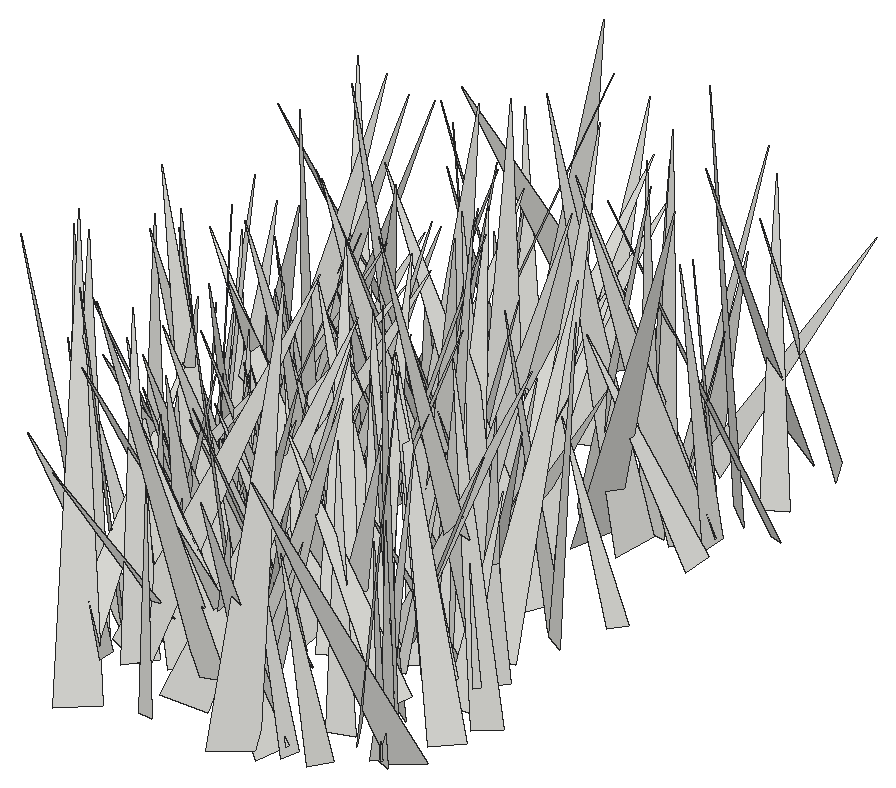
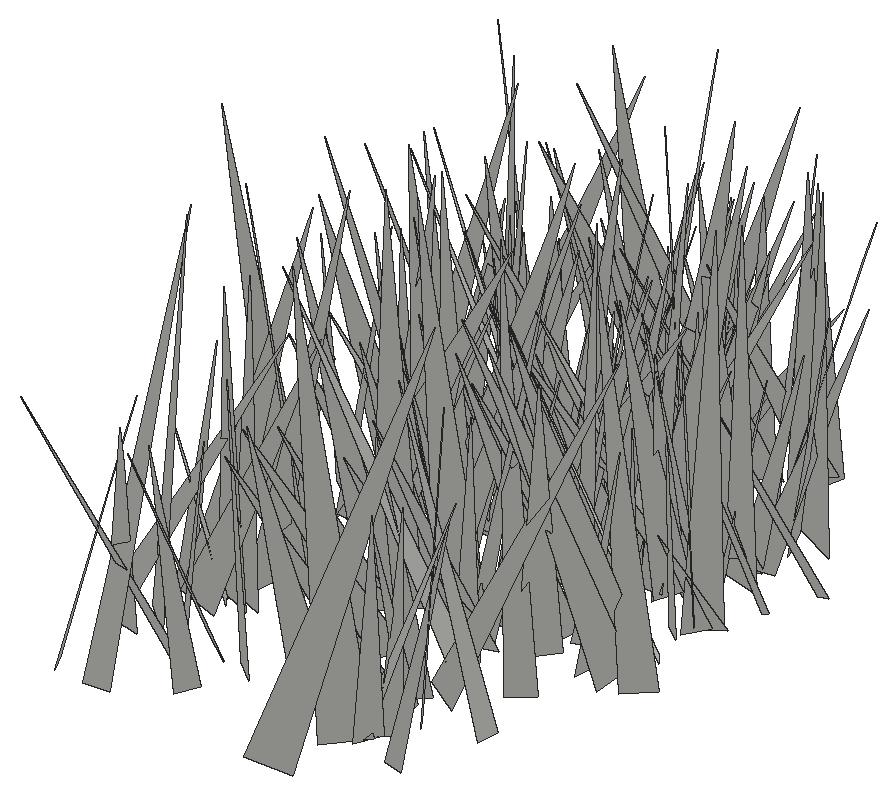
# SketchUp Ruby script. Lengths in inches.
U = 1.inch
M = Sketchup.active_model
def pt(a) = Geom::Point3d.new(a.map { |v| v * U })
def face(e, loops, mat)
  f = e.add_face(loops[0].map { |a| pt(a) })
  loops[1..].each { |l| e.add_face(l.map { |a| pt(a) }).erase! }
  f.material = f.back_material = mat if mat
  f
end
# faces: each face lists its corners as indices into pts; further lists are holes
def faces(e, pts, list, mat = nil) = list.each { |f| face(e, (f[0].is_a?(Array) ? f : [f]).map { |l| l.map { |i| pts[i] } }, mat) }
# xy, xz, yz: faces in a plane at the given z, y or x. An outline is a flat list of corners, or four numbers for a rectangle; further outlines are holes
def ring(l) = l.size == 4 ? [[l[0], l[1]], [l[2], l[1]], [l[2], l[3]], [l[0], l[3]]] : l.each_slice(2).to_a
def flat(e, list, mat, &to3) = list.each { |f| face(e, (f[0].is_a?(Array) ? f : [f]).map { |l| ring(l).map { |u, v| to3.(u, v) } }, mat) }
def xy(e, z, list, mat = nil) = flat(e, list, mat) { |x, y| [x, y, z] }
def xz(e, y, list, mat = nil) = flat(e, list, mat) { |x, z| [x, y, z] }
def yz(e, x, list, mat = nil) = flat(e, list, mat) { |y, z| [x, y, z] }
def lines(e, pts, list) = list.each { |a, b| e.add_line(pt(pts[a]), pt(pts[b])) }
# prism: a flat outline (further loops are holes) pulled along v
def prism(e, loops, v, mat = nil)
  f = face(e, loops, mat); d = Geom::Vector3d.new(v.map { |x| x * U })
  f.pushpull(f.normal.samedirection?(d) ? d.length : -d.length)
end
def box(e, o, s, mat = nil) = prism(e, [[o, [o[0] + s[0], o[1], o[2]], [o[0] + s[0], o[1] + s[1], o[2]], [o[0], o[1] + s[1], o[2]]]], [0, 0, s[2]], mat)
def at(x, y, z, deg = 0) = Geom::Transformation.translation(pt([x, y, z])) * Geom::Transformation.rotation(ORIGIN, Z_AXIS, deg.degrees)
def axes(o, x, y, z) = Geom::Transformation.new([*x, 0, *y, 0, *z, 0, *pt(o).to_a, 1])
def part(name) = M.definitions.add(name)
# library, detail: a bought-in or finely detailed component or shape, given as its bounding box
def library(name, o, s) = part(name).tap { |d| box(d.entities, o, s) }
def detail(e, o, s) = box(e.add_group.entities, o, s)
def put(e, d, t, mat = nil) = e.add_instance(d, t).tap { |i| i.material = mat if mat }
def group(e, t, mat = nil) = e.add_group.tap { |g| g.transformation = t; g.material = mat if mat }.entities
root = M.entities
c1 = part("fur_instance\#9")
p = [[0.8125,0,1.79],[0.67,-0.02,1.48],[0,-0.11,0],[0,0.11,0]]
faces(c1.entities,p,[[0,1,2,3]])
put(root,c1,axes([99.53,207.82,-27.1],[-3.854,-0.48704,1.31581],[-0.33639,4.05498,0.51565],[1.36213,-0.37663,3.85028]))
put(root,c1,axes([100.16,194.93,-28.22],[1.87849,6.8023,2.53671],[7.02619,-2.36292,1.13321],[-1.82724,-2.09291,6.96533]))
put(root,c1,axes([100.67,195.38,-28.22],[-4.99068,-1.45127,1.21381],[-1.71677,4.91279,-1.18474],[0.79513,1.49823,5.06058]))
put(root,c1,axes([99.54,205.16,-28.22],[2.36348,3.65871,1.87372],[3.9267,-2.64879,0.21906],[-1.21573,-1.4425,4.3502]))
put(root,c1,axes([102.27,193.58,-27.1],[-6.74391,-2.32387,0.77011],[-2.44649,6.31426,-2.37034],[-0.09,2.49068,6.72772]))
put(root,c1,axes([98.67,206.66,-27.1],[6.0321,-2.57805,3.10449],[-3.62742,-5.91038,2.14001],[-1.76807,3.33038,6.20104]))
put(root,c1,axes([97.26,207.74,-27.1],[1.41766,-6.83451,0.48866],[-6.53171,-1.19719,2.20513],[2.07029,0.90294,6.62252]))
put(root,c1,axes([98.46,207.52,-27.1],[6.56769,-0.93589,1.93904],[-1.50422,-6.44796,1.98276],[-1.54048,2.30611,6.3308]))
put(root,c1,axes([99.47,201.66,-28.22],[6.10585,-2.9623,2.45846],[-2.96929,-6.55789,-0.52733],[-2.45002,0.56525,6.76598]))
put(root,c1,axes([101.33,207.83,-27.1],[-5.19034,4.80556,0.45379],[4.78626,5.21014,-0.43029],[0.62529,0.00866,7.0603]))
put(root,c1,axes([100.43,197.4,-28.22],[3.46257,-3.0651,1.27719],[-2.41097,-3.5895,-2.07802],[-2.28326,-0.85797,4.13111]))
put(root,c1,axes([102.11,211.93,-27.1],[-3.14306,-6.22127,0.26286],[-6.12359,3.03481,-1.39417],[-1.12913,0.859,6.8293]))
put(root,c1,axes([100.4,198.49,-28.22],[1.00735,6.64791,2.58508],[7.07427,-1.26504,0.49655],[-0.91221,-2.46923,6.70544]))
put(root,c1,axes([100.78,197.67,-28.22],[-2.91756,2.69263,1.56889],[3.08399,2.80363,0.92331],[0.448,-1.76443,3.86133]))
put(root,c1,axes([100.94,194.41,-27.1],[-0.82841,6.75025,1.93378],[7.00258,0.65031,0.72978],[-0.51887,-2.00072,6.76162]))
put(root,c1,axes([100.41,216.59,-27.1],[-1.40933,-4.17013,0.64925],[-4.20295,1.44894,0.18319],[0.38311,0.55526,4.39803]))
put(root,c1,axes([100.12,202.41,-28.22],[2.1369,3.02619,1.55246],[3.28055,-2.31782,0.00255],[-0.89775,-1.26656,3.70461]))
put(root,c1,axes([101.0625,199.84,-28.22],[2.9038,6.51052,1.10748],[6.2299,-3.10193,1.9005],[-2.1913,-0.1914,6.87074]))
put(root,c1,axes([100.12,201.24,-28.22],[-3.74017,-2.83655,2.38458],[-3.12746,4.23356,0.13062],[1.98777,1.32365,4.69232]))
put(root,c1,axes([102.41,191.93,-28.22],[-7.32021,3.8589,0.48336],[3.73123,7.2592,-1.44642],[1.09666,1.05977,8.14767]))
put(root,c1,axes([100.45,201.95,-27.1],[-4.55508,3.55475,2.05706],[3.40532,4.98624,-1.07596],[2.29598,-0.34303,5.67691]))
put(root,c1,axes([101.89,200.34,-28.22],[-5.70534,2.42628,0.74712],[2.22137,5.6608,-1.42016],[1.22905,1.03174,6.03498]))
put(root,c1,axes([100.52,199.53,-28.22],[-3.02452,-1.82217,1.01563],[-1.34667,3.07159,1.50047],[1.5932,-0.86291,3.19635]))
put(root,c1,axes([102.8,214.93,-27.1],[-4.27144,-3.27285,0.83505],[-3.36103,3.98484,-1.57435],[-0.33515,1.75031,5.14569]))
put(root,c1,axes([100.61,198.03,-28.22],[-0.48959,-3.44443,1.08487],[-3.54488,0.6673,0.51889],[0.68909,0.98557,3.44014]))
put(root,c1,axes([98.13,205.59,-27.1],[4.83025,3.81866,0.07193],[3.65702,-4.5907,-1.86288],[1.10161,-1.50398,5.86882]))
put(root,c1,axes([101.55,195.35,-27.1],[-4.35453,-4.53446,2.05004],[-4.74623,4.60317,0.10013],[1.49574,1.4055,6.28595]))
put(root,c1,axes([100.39,206.33,-27.1],[5.08436,-3.96797,0.13679],[-3.71243,-4.83007,-2.12193],[-1.40762,-1.5937,6.0904]))
put(root,c1,axes([100.04,205.7,-27.1],[7.02888,1.27959,1.54515],[0.73768,-6.88381,2.34499],[-1.86566,2.099,6.7486]))
put(root,c1,axes([101.61,201.23,-27.1],[2.47706,-6.70826,1.39737],[-6.69174,-2.68793,-1.04158],[-1.47445,0.92925,7.07472]))
put(root,c1,axes([99.2,206.34,-27.1],[-0.29614,5.30233,1.4786],[4.87042,0.94241,-2.40408],[2.56516,-1.17721,4.73528]))
put(root,c1,axes([102.18,215.67,-27.1],[-4.07522,2.66076,1.05763],[2.66001,4.19896,-0.31421],[1.05952,-0.30776,4.85678]))
put(root,c1,axes([98.56,199.53,-28.22],[3.67258,4.04026,0.63824],[3.75616,-2.99162,-2.6759],[1.61937,-2.22383,4.75932]))
put(root,c1,axes([97.76,197.5,-28.22],[4.06376,5.39951,0.02576],[4.83357,-3.62337,-3.0294],[2.40665,-1.8401,6.04083]))
put(root,c1,axes([101.64,213.56,-27.1],[-4.27511,-3.26782,2.05551],[-3.38668,4.64678,0.34365],[1.85313,0.95347,5.37002]))
put(root,c1,axes([102.23,204.49,-28.22],[-3.60643,-6.53276,3.39182],[-7.2869,3.70246,-0.61691],[1.0404,3.28673,7.43658]))
put(root,c1,axes([99.24,213.11,-27.1],[6.07626,0.90493,0.17774],[0.92213,-5.94508,-1.25588],[0.01299,-1.26833,6.01354]))
put(root,c1,axes([100.4375,198.77,-27.1],[2.54415,-5.74451,1.38415],[-5.89364,-2.3587,1.04378],[0.42454,1.68081,6.19537]))
put(root,c1,axes([102.03,200.9,-27.1],[3.56835,-1.26097,2.05366],[-1.59686,-3.9854,0.32755],[-1.80488,1.03305,3.77039]))
put(root,c1,axes([105.05,198.42,-28.22],[-4.54236,-5.48641,0.31776],[-5.31376,4.27953,-2.06985],[-1.40202,1.55551,6.81539]))
put(root,c1,axes([101.58,192.82,-27.1],[-1.51981,5.35977,0.02073],[5.22969,1.48762,-1.21441],[1.17387,0.31183,5.43711]))
put(root,c1,axes([102.57,200.48,-27.1],[3.27442,-5.47757,0.11686],[-5.10679,-3.10069,-2.24625],[-1.98447,-1.05885,5.97327]))
put(root,c1,axes([100.9375,203.56,-27.1],[2.11868,-4.0714,0.72457],[-4.11944,-2.00647,0.77101],[0.3627,0.99394,4.52445]))
put(root,c1,axes([101.58,200.22,-27.1],[3.83893,-0.81047,1.08867],[-0.8917,-3.9684,0.19003],[-1.0232,0.41758,3.91895]))
put(root,c1,axes([101.18,202.21,-27.1],[-2.08812,-6.42397,1.05341],[-6.15561,2.30841,1.87538],[2.11792,0.37569,6.48927]))
put(root,c1,axes([101.77,215.03,-27.1],[3.2467,-2.02133,0.75684],[-1.94033,-3.33216,-0.57574],[-0.94537,-0.10279,3.78092]))
put(root,c1,axes([103.27,203.58,-27.1],[-3.89447,-3.70378,1.65585],[-4.00703,3.87088,-0.766],[0.63525,1.71028,5.3196]))
put(root,c1,axes([102.22,213.4375,-27.1],[3.63401,0.67625,1.41653],[0.37628,-3.84346,0.86953],[-1.5239,0.6636,3.59267]))
put(root,c1,axes([101.24,199.92,-28.22],[5.91646,3.40669,0.5347],[3.12979,-5.75065,2.00759],[-1.44773,1.49011,6.52531]))
put(root,c1,axes([101.53,197.16,-28.22],[-0.19463,-4.95849,1.24268],[-5.00803,0.4343,0.94858],[1.02496,1.18047,4.8708]))
put(root,c1,axes([104.27,207.44,-27.1],[-7.25051,-1.24633,1.39987],[-1.43303,7.2913,-0.93068],[1.20805,1.16894,7.29774]))
put(root,c1,axes([99.125,201.36,-28.22],[2.23337,6.49328,0.05356],[5.9184,-2.0122,-2.84202],[2.67172,-0.9705,6.25089]))
put(root,c1,axes([100.08,210.36,-27.1],[-0.39765,-7.51588,0.89638],[-7.02687,0.7002,2.75371],[2.81337,0.68655,7.00455]))
put(root,c1,axes([104.01,203.61,-27.1],[-0.12405,-5.8754,2.10648],[-6.00776,-0.4589,-1.63376],[-1.69244,2.05962,5.64504]))
put(root,c1,axes([104.07,198.35,-28.22],[0.25275,3.74041,1.98428],[3.79537,-1.08135,1.55493],[-1.87703,-1.68284,3.41127]))
put(root,c1,axes([103.41,193.92,-27.1],[-5.08391,3.17186,1.29588],[3.17676,5.23223,-0.34381],[1.28383,-0.38638,5.98237]))
put(root,c1,axes([102.92,197.95,-27.1],[-0.42877,3.87256,1.55947],[4.17346,0.35848,0.25729],[-0.1042,-1.57711,3.88772]))
put(root,c1,axes([104.36,197.49,-27.1],[-1.56968,-5.60909,0.11931],[-5.50885,1.51747,-1.1357],[-1.06238,0.41882,5.71278]))
put(root,c1,axes([106.45,200.89,-27.1],[-3.37764,5.82202,0.02709],[5.22944,3.02002,2.9728],[-2.55923,-1.51283,6.03878]))
put(root,c1,axes([104.73,196.54,-27.1],[-3.07753,7.46975,2.03134],[7.70521,2.74591,1.57617],[-0.74375,-2.46119,7.92363]))
put(root,c1,axes([103.76,198.47,-28.22],[-4.72142,-2.258,0.83052],[-2.14472,4.77905,0.80066],[1.09019,-0.37724,5.17198]))
put(root,c1,axes([104.77,194.54,-27.1],[-1.73609,5.26171,0.91511],[5.1615,1.40586,1.70864],[-1.37182,-1.3693,5.27069]))
put(root,c1,axes([101.43,206.43,-27.1],[5.10289,-1.83511,1.25864],[-2.13691,-4.91957,1.49087],[-0.62081,1.84972,5.21387]))
put(root,c1,axes([105.28,195.8,-28.22],[-0.91918,-4.72146,0.08029],[-4.18667,0.777,-2.23865],[-2.18412,0.49761,4.25741]))
put(root,c1,axes([103.34,208.12,-27.1],[-1.39577,-4.42794,0.41329],[-4.44248,1.40819,0.08395],[0.20461,0.36877,4.64196]))
put(root,c1,axes([101.45,199.2,-28.22],[4.36053,2.62617,0.62372],[2.69593,-4.29581,-0.7602],[-0.13318,-0.97427,5.03319]))
put(root,c1,axes([101.8,207.12,-27.1],[3.71055,0.76796,0.33165],[0.80764,-3.68168,-0.51076],[-0.21789,-0.56867,3.7546]))
put(root,c1,axes([103.62,219.07,-27.1],[3.75973,-6.87339,0.18092],[-6.4988,-3.61971,-2.46477],[-2.2454,-1.03249,7.43666]))
put(root,c1,axes([102.93,198.07,-28.22],[5.9616,4.7587,3.0284],[5.08757,-6.43918,0.10304],[-2.43578,-1.80245,7.62727]))
put(root,c1,axes([102.84,195.16,-27.1],[4.75143,0.92242,1.33841],[0.70934,-4.89704,0.85681],[-1.46255,0.62163,4.7637]))
put(root,c1,axes([102.83,209.74,-27.1],[3.43508,-2.31671,0.74566],[-2.27877,-3.51457,-0.42176],[-0.85461,0.05948,4.12177]))
put(root,c1,axes([103.88,198.78,-28.22],[1.78326,-6.33726,0.7797],[-6.26284,-1.89367,-1.06754],[-1.24322,0.44943,6.49625]))
put(root,c1,axes([103.3,197.05,-27.1],[2.16413,-4.87719,1.14426],[-4.95965,-2.26151,-0.2591],[-0.70577,0.93721,5.32947]))
put(root,c1,axes([104.68,199.7,-28.22],[2.20766,-6.15742,1.48059],[-5.96151,-2.54967,-1.71445],[-2.13691,0.75174,6.31254]))
put(root,c1,axes([104.7,195.52,-28.22],[-3.64875,-2.02244,1.121],[-2.25149,3.58457,-0.86132],[0.52696,1.3118,4.08188]))
put(root,c1,axes([103.02,208.6,-27.1],[-0.26942,5.43204,0.24352],[5.36362,0.30555,-0.88154],[0.89325,-0.19629,5.36679]))
put(root,c1,axes([104.49,192.81,-28.22],[1.15906,3.62365,1.13013],[3.60388,-1.42153,0.86183],[-1.19166,-0.77453,3.7056]))
put(root,c1,axes([102.61,212.53,-27.1],[1.94389,-4.04886,0.80465],[-4.08173,-1.75236,1.04312],[0.61659,1.16421,4.36851]))
put(root,c1,axes([104.93,201.1,-28.22],[-5.52274,-3.05851,1.02558],[-2.84433,5.57616,1.31266],[1.52186,-0.67738,6.17511]))
put(root,c1,axes([103.68,202.9,-27.1],[3.85077,0.95797,1.10657],[0.6489,-3.90916,1.12606],[-1.31192,0.87829,3.80501]))
put(root,c1,axes([103.48,200.92,-27.1],[-2.78361,3.37072,1.19614],[3.02117,3.0272,-1.49988],[1.91443,0.12385,4.10617]))
put(root,c1,axes([103.35,209.32,-27.1],[-3.61899,-3.55384,3.43713],[-4.24844,4.41399,0.09065],[2.52873,2.32973,5.07136]))
put(root,c1,axes([105.98,194.57,-27.1],[-1.13695,-6.80591,1.9758],[-6.92615,0.64332,-1.76957],[-1.50086,2.18691,6.66945]))
put(root,c1,axes([102.68,216.23,-27.1],[5.49312,-5.94068,1.74056],[-6.16398,-5.4638,0.80479],[-0.57141,1.8305,8.05098]))
put(root,c1,axes([105.45,199.26,-27.1],[-1.01525,-4.25558,0.24661],[-4.20456,0.95799,-0.77812],[-0.70176,0.41691,4.30525]))
put(root,c1,axes([103.39,206.96,-27.1],[5.19652,-2.78136,0.42044],[-2.54268,-5.02221,-1.79688],[-1.20313,-1.39929,5.61347]))
put(root,c1,axes([104.83,197.23,-27.1],[-2.5051,-3.46967,0.23869],[-3.39401,2.50314,0.76559],[0.75915,-0.25846,4.21047]))
put(root,c1,axes([105.66,200.01,-27.1],[-2.79772,3.91125,0.86225],[4.00509,2.73873,0.57209],[0.02536,-1.03446,4.77471]))
put(root,c1,axes([105.96,207.42,-27.1],[-3.1075,-6.9448,0.74353],[-6.98342,3.07514,-0.46373],[-0.12218,0.86773,7.5942]))
put(root,c1,axes([102.39,210.39,-27.1],[7.40183,3.33475,0.3809],[3.31775,-7.40888,0.39208],[-0.5081,0.20159,8.10888]))
put(root,c1,axes([104.03,208.39,-27.1],[-3.12669,6.25889,3.83958],[6.87271,3.96367,-0.86451],[2.58493,-2.9678,6.9428]))
put(root,c1,axes([105.55,201.92,-28.22],[-3.08604,-1.58363,1.00431],[-1.62158,3.22493,0.10239],[0.94181,0.36349,3.46714]))
put(root,c1,axes([106.84,198.65,-27.1],[-4.54566,0.43172,0.55069],[0.54174,4.46219,0.97364],[0.44289,-1.02717,4.4611]))
put(root,c1,axes([102.85,194.11,-27.1],[1.48421,7.77893,1.22221],[7.56365,-1.06243,-2.42301],[2.19017,-1.60247,7.53948]))
put(root,c1,axes([109.28,193.46,-28.22],[-2.18408,5.95276,0.46734],[5.01759,1.55993,3.57972],[-3.2369,-1.59851,5.23366]))
put(root,c1,axes([102.64,199.72,-27.1],[1.86343,6.88556,0.79652],[6.51007,-1.45535,-2.64927],[2.37997,-1.41024,6.62304]))
put(root,c1,axes([105.21,206.23,-27.1],[4.98467,2.72403,1.68688],[2.57744,-5.26236,0.88159],[-1.90334,0.00786,5.61161]))
put(root,c1,axes([106.95,194.92,-27.1],[-6.4254,-4.61842,2.37343],[-5.01235,6.50279,-0.91585],[1.35622,2.15235,7.85982]))
put(root,c1,axes([104.47,201.32,-28.22],[4.44163,5.80553,0.93246],[5.82565,-4.50337,0.28854],[-0.79717,-0.56325,7.30404]))
put(root,c1,axes([105.65,214.26,-27.1],[-4.4871,3.83069,1.41429],[3.5666,4.69982,-1.41404],[1.98841,0.2144,5.72789]))
put(root,c1,axes([105.81,200.99,-28.22],[-0.46017,-7.01963,1.64197],[-7.20868,0.46604,-0.02793],[0.07879,1.64032,7.03464]))
put(root,c1,axes([104.03,197.22,-27.1],[3.98681,-3.04122,0.56389],[-3.08769,-3.85909,1.01744],[0.18196,1.14894,4.91004]))
put(root,c1,axes([105.97,199.24,-28.22],[-2.87377,-5.9267,0.11201],[-5.79461,2.83495,1.33509],[1.24935,-0.48389,6.44995]))
put(root,c1,axes([104.33,212.59,-27.1],[-1.05033,5.0969,0.69056],[4.61293,1.24522,-2.17458],[2.27512,-0.17172,4.72788]))
put(root,c1,axes([105.11,210.84,-27.1],[-2.16647,5.60636,0.16983],[5.26617,2.09582,-2.00715],[1.93067,0.57445,5.66535]))
put(root,c1,axes([107.71,204.57,-27.1],[2.58278,-6.81445,2.81399],[-6.72051,-3.40212,-2.07037],[-3.03151,1.73634,6.98721]))
put(root,c1,axes([106.48,196.6,-28.22],[2.5877,-3.76016,0.15432],[-3.53923,-2.49522,-1.45139],[-1.27925,-0.70276,4.32764]))
put(root,c1,axes([105.9375,196.74,-28.22],[4.8135,2.02359,1.54657],[1.94555,-5.05552,0.55956],[-1.64367,-0.05793,5.19149]))
put(root,c1,axes([104.54,196.76,-28.22],[6.50661,-0.43072,0.76621],[-0.39332,-6.54513,-0.33931],[-0.78607,-0.29036,6.51202]))
put(root,c1,axes([107.4375,197.33,-27.1],[-4.91949,-2.25789,1.34677],[-2.33985,5.06309,-0.05864],[1.19873,0.61667,5.41258]))
put(root,c1,axes([108.43,200.8,-28.22],[-3.37701,5.49526,1.43426],[5.6473,3.0721,1.52623],[-0.60248,-2.00587,6.26679]))
put(root,c1,axes([105.73,195.26,-27.1],[2.79472,-2.37927,0.19168],[-2.37504,-2.80125,-0.14262],[-0.23842,0.01542,3.66757]))
put(root,c1,axes([106.1,206.95,-27.1],[4.26152,0.65659,1.09682],[0.47447,-4.35714,0.76482],[-1.18701,0.6156,4.24343]))
put(root,c1,axes([104.97,194.25,-28.22],[-3.36255,6.42423,2.20976],[5.77924,4.00105,-2.8377],[3.57129,-0.42595,6.67271]))
put(root,c1,axes([108.16,198.3,-27.1],[-2.69969,6.39263,0.77147],[6.43614,2.65406,0.5304],[-0.19237,-0.91623,6.91901]))
put(root,c1,axes([106.88,208.33,-27.1],[4.92232,-5.34816,3.43981],[-5.97476,-5.37881,0.1869],[-2.17654,2.67018,7.26616]))
put(root,c1,axes([108.22,204.24,-27.1],[-4.1053,-4.23157,0.31859],[-4.21802,4.11764,0.33835],[0.46467,-0.00766,5.88602]))
put(root,c1,axes([111.23,204.73,-27.1],[-3.57057,6.8988,1.02898],[6.50769,2.8788,3.28081],[-2.51043,-2.34953,7.04122]))
put(root,c1,axes([108.18,200.41,-27.1],[2.13883,-4.28297,3.06723],[-5.00629,-2.68295,-0.2554],[-1.63976,2.60467,4.7805]))
put(root,c1,axes([107.53,195.35,-28.22],[1.37303,-5.10418,0.31363],[-5.09334,-1.39399,-0.38851],[-0.45708,0.20095,5.27134]))
put(root,c1,axes([106.73,205.19,-28.22],[6.65936,-3.07974,1.86174],[-3.09449,-6.89952,-0.34452],[-1.83712,0.458,7.32893]))
put(root,c1,axes([106.79,196,-27.1],[3.4607,5.10853,1.2476],[5.25066,-3.43918,-0.48234],[-0.29016,-1.30574,6.15149]))
put(root,c1,axes([107.52,208.44,-27.1],[-1.55041,4.4226,0.08121],[4.26043,1.51619,-1.23272],[1.18941,0.33394,4.52145]))
put(root,c1,axes([106.1875,196.55,-28.22],[4.99795,-3.82327,1.26682],[-4.01963,-4.86241,1.18375],[-0.25457,1.71502,6.18026]))
put(root,c1,axes([109.75,204.97,-27.1],[-3.22494,-3.97651,0.65226],[-4.0077,3.07801,-1.05003],[-0.42001,1.16258,5.01102]))
put(root,c1,axes([108.18,192.79,-28.22],[5.95771,-4.00613,4.25574],[-5.13988,-6.48421,1.09155],[-2.78246,3.40011,7.09591]))
put(root,c1,axes([109.43,201.05,-28.22],[-1.2405,4.10694,0.41743],[4.03089,1.11105,1.04764],[-0.89058,-0.69186,4.16031]))
put(root,c1,axes([108.11,204.12,-27.1],[-3.37958,0.77927,1.41196],[0.41341,3.58754,-0.99047],[1.55884,0.73803,3.32382]))
put(root,c1,axes([108.17,214.62,-27.1],[3.30572,4.13092,2.03155],[4.38871,-3.58299,0.14433],[-1.38957,-1.489,5.28881]))
put(root,c1,axes([108.15,200.93,-27.1],[3.13012,3.09581,1.75638],[3.35561,-3.34662,-0.08138],[-1.18695,-1.29717,4.40172]))
put(root,c1,axes([109.8125,193.71,-28.22],[-4.0966,0.35691,0.30901],[0.31396,4.07547,-0.54495],[0.35257,0.51784,4.07585]))
put(root,c1,axes([107.12,199.87,-27.1],[5.77926,4.78065,0.80242],[4.74367,-5.8345,0.5954],[-0.99801,-0.04845,7.47663]))
put(root,c1,axes([109.32,198.22,-27.1],[-1.91608,6.79372,1.10059],[6.8739,1.94553,-0.04218],[0.33984,-1.04766,7.05863]))
put(root,c1,axes([106.38,200.84,-27.1],[5.98331,3.57339,0.75673],[3.63565,-5.68637,-1.89446],[0.35186,-2.00943,6.70672]))
put(root,c1,axes([107.81,199.1,-27.1],[2.67886,-4.09104,0.57639],[-4.11516,-2.58128,0.80469],[0.36641,0.91951,4.82342]))
put(root,c1,axes([109.16,201.91,-28.22],[-5.34624,-2.21651,3.3319],[-3.00843,5.89263,-0.90721],[2.6389,2.22728,5.71596]))
put(root,c1,axes([111.65,196.98,-27.1],[-4.58774,2.19144,0.09862],[2.15217,4.45217,1.18567],[-0.42461,-1.11142,4.94408]))
put(root,c1,axes([109.84,214.01,-27.1],[2.78013,5.13783,0.11647],[4.85085,-2.66723,1.86951],[-1.69707,0.79284,5.53456]))
put(root,c1,axes([110.23,195.85,-28.22],[-0.93822,4.8343,1.08723],[4.93478,0.81164,0.64956],[-0.44769,-1.18472,4.88147]))
put(root,c1,axes([111.18,209.96,-27.1],[-8.03417,0.61584,1.78735],[0.70083,8.21761,0.3188],[1.75577,-0.4621,8.05143]))
put(root,c1,axes([112.21,212.03,-27.1],[-0.7555,-5.85213,2.53673],[-5.87032,-0.36099,-2.58111],[-2.49433,2.62211,5.30623]))
put(root,c1,axes([110.76,205,-27.1],[0.70826,8.01559,0.32411],[7.89046,-0.75477,1.42384],[-1.44754,-0.19233,7.91985]))
put(root,c1,axes([108.82,216.8,-27.1],[3.79566,-1.87078,0.73995],[-1.92959,-3.83243,0.2087],[-0.56925,0.51676,4.2265]))
put(root,c1,axes([110.46,198.67,-27.1],[1.53322,3.39,0.04746],[3.12816,-1.43461,1.41479],[-1.30727,0.54307,3.44111]))
put(root,c1,axes([110.29,200.85,-28.22],[2.96295,7.07925,2.39249],[7.30087,-3.29107,0.69644],[-1.59283,-1.91622,7.64263]))
put(root,c1,axes([110.62,214.79,-27.1],[-2.70575,-2.79772,1.42447],[-3.05403,2.78134,-0.3384],[0.7275,1.27058,3.87735]))
put(root,c1,axes([108.43,203.74,-27.1],[2.40948,7.1196,1.80641],[7.28749,-2.07931,-1.52526],[0.91887,-2.17835,7.35989]))
put(root,c1,axes([111.09,200.8,-28.22],[-5.51425,5.90533,1.65371],[5.90522,5.71303,-0.71018],[1.6541,-0.70927,8.04832]))
put(root,c1,axes([112.04,200.62,-28.22],[-1.30366,-3.70433,0.26528],[-3.50778,1.13584,-1.37745],[-1.21983,0.69265,3.67753]))
put(root,c1,axes([112.16,201.13,-27.1],[-1.47229,-7.46087,2.3597],[-7.72207,0.99683,-1.66627],[-1.2659,2.59656,7.41996]))
put(root,c1,axes([110.82,198.17,-28.22],[3.12486,4.78234,3.10342],[5.39282,-3.6275,0.15986],[-1.8492,-2.49745,5.71052]))
put(root,c1,axes([111.7,199.15,-27.1],[-2.10663,5.00928,1.58804],[5.23429,1.84857,1.1125],[-0.46582,-1.88217,5.31913]))
put(root,c1,axes([111.03,211.02,-27.1],[1.52535,6.05061,2.3847],[6.37233,-1.8801,0.69429],[-1.30004,-2.1163,6.20117]))
put(root,c1,axes([110.96,193.86,-28.22],[2.35364,-2.97334,1.61897],[-3.0072,-2.74184,-0.66374],[-1.55518,0.80187,3.73361]))
put(root,c1,axes([108.58,205.67,-27.1],[4.05513,-1.76427,0.28786],[-1.75227,-3.78191,1.50543],[0.35366,1.49134,4.15818]))
put(root,c1,axes([110.79,202.9,-27.1],[-3.9364,0.91485,1.26316],[0.41585,3.92071,-1.54367],[1.50319,1.31107,3.73488]))
put(root,c1,axes([111.45,211.15,-27.1],[1.52535,6.57132,1.88983],[6.63248,-1.89273,1.22809],[-1.66251,-1.52175,6.63331]))
put(root,c1,axes([108.83,210.11,-27.1],[5.37674,4.78999,2.15375],[5.23773,-5.117,-1.69543],[-0.38579,-2.71372,6.99849]))
put(root,c1,axes([113.3,199.85,-27.1],[-7.7657,1.30292,0.44128],[1.14319,7.51969,-2.08465],[0.76515,1.98873,7.59328]))
put(root,c1,axes([109.67,202.19,-27.1],[4.18382,1.92252,0.07247],[1.86113,-4.08842,1.01327],[-0.48737,0.89131,4.49152]))
put(root,c1,axes([109.6,200.125,-27.1],[4.10602,0.97464,0.35289],[0.9844,-4.11806,-0.08026],[-0.32469,-0.15985,4.21935]))
put(root,c1,axes([113.375,197.45,-28.22],[-1.94953,6.2532,0.70862],[6.08536,1.68405,1.8809],[-1.60411,-1.2111,6.27419]))
put(root,c1,axes([111.65,196.67,-27.1],[-3.98091,-5.38333,3.048],[-6.04161,4.16252,-0.53901],[1.33021,2.79489,6.67363]))
put(root,c1,axes([112.32,204.38,-27.1],[-5.31437,-1.63311,1.48269],[-1.72892,5.48589,-0.1545],[1.36976,0.58821,5.55749]))
put(root,c1,axes([114.45,213.24,-27.1],[-3.99389,-5.07881,0.29207],[-4.86869,3.70838,-2.09153],[-1.47493,1.51142,6.11318]))
put(root,c1,axes([112.26,195.27,-28.22],[-4.99347,0.21503,1.45697],[-0.36457,4.80955,-1.95935],[1.42691,1.98134,4.59803]))
put(root,c1,axes([112.45,211.38,-27.1],[3.31279,-6.01066,2.01721],[-5.81791,-3.7865,-1.72802],[-2.51972,0.84034,6.64203]))
put(root,c1,axes([109.78,204.02,-27.1],[4.97063,-0.22915,0.23226],[-0.15729,-4.7897,-1.3593],[-0.28585,-1.34904,4.78665]))
put(root,c1,axes([108.97,200.44,-27.1],[3.86219,5.07234,0.99731],[5.04282,-3.42294,-2.11973],[1.1372,-2.04809,6.01264]))
put(root,c1,axes([112.39,195.59,-28.22],[-4.80095,-0.85986,1.55653],[-1.24807,4.82151,-1.18603],[1.26668,1.49164,4.73094]))
put(root,c1,axes([113.22,214.71,-27.1],[-0.43332,5.55714,0.38235],[5.39105,0.32188,1.43136],[-1.40165,-0.47995,5.3871]))
put(root,c1,axes([113.78,199.03,-28.22],[-0.60049,6.11637,0.8715],[5.86899,0.29123,2.00004],[-1.92986,-1.0175,5.81123]))
put(root,c1,axes([113.5,210.33,-27.1],[-4.40105,0.97982,0.44244],[1.06612,4.21791,1.26401],[0.13855,-1.33202,4.328]))
put(root,c1,axes([112.53,213.69,-27.1],[-4.94486,-5.49387,2.91837],[-6.02867,5.15162,-0.51692],[1.53451,2.53562,7.37341]))
put(root,c1,axes([113.17,195.68,-28.22],[1.05272,-6.58483,0.46236],[-6.33643,-1.13928,-1.79827],[-1.85027,0.15508,6.42141]))
put(root,c1,axes([112.53,195.15,-28.22],[1.66971,3.21733,1.57549],[3.35444,-2.01427,0.55833],[-1.25742,-1.10127,3.58153]))
put(root,c1,axes([111.65,211.23,-27.1],[2.95559,2.2846,0.71516],[2.24296,-3.03986,0.44126],[-0.83663,-0.07885,3.70947]))
put(root,c1,axes([111.85,201.5,-28.22],[-4.58199,0.67037,2.42399],[0.81188,5.16228,0.10702],[2.38033,-0.47034,4.62953]))
put(root,c1,axes([111.27,218.46,-27.1],[-2.73458,-7.67612,0.26637],[-7.34259,2.69559,2.30041],[2.25392,-0.53168,7.81722]))
put(root,c1,axes([109.74,215.85,-27.1],[2.70061,4.81345,0.08968],[4.52857,-2.505,-1.92033],[1.63383,-1.01307,5.17446]))
put(root,c1,axes([112.31,201.24,-27.1],[-4.09876,5.0884,1.14662],[4.86258,4.25523,-1.50159],[1.8873,0.0873,6.359]))
put(root,c1,axes([112.13,199.5,-28.22],[-0.72601,3.76819,0.7458],[3.80081,0.81458,-0.41575],[0.55615,-0.64789,3.8149]))
put(root,c1,axes([113.08,211.65,-27.1],[-4.88413,-0.13594,1.40409],[-0.16648,5.08029,-0.08723],[1.4008,0.12978,4.88524]))
put(root,c1,axes([113.28,217.97,-27.1],[-4.38014,-2.49103,0.91186],[-2.44951,4.47381,0.4553],[1.01814,0.04674,5.01832]))
put(root,c1,axes([109.81,209.55,-27.1],[8.0282,-2.33719,0.44231],[-2.30718,-8.02996,-0.55383],[-0.57877,-0.40914,8.34313]))
put(root,c1,axes([111.95,194.65,-27.1],[5.69134,3.55142,2.30083],[3.82093,-5.97012,-0.23634],[-1.81848,-1.42926,6.70433]))
put(root,c1,axes([114.0625,205.46,-27.1],[-1.40668,3.30295,0.84871],[3.29754,1.08331,1.24951],[-0.86952,-1.23511,3.36556]))
put(root,c1,axes([113.125,203.34,-27.1],[2.73063,4.59292,1.67983],[4.59916,-3.06583,0.90635],[-1.66266,-0.93747,5.2659]))
